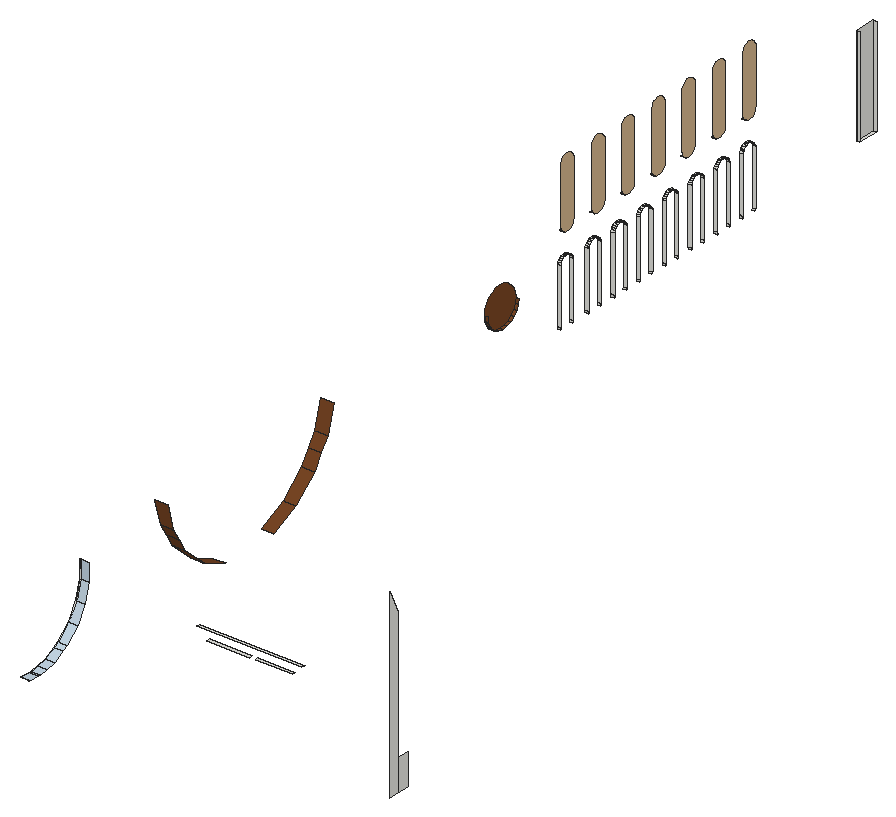
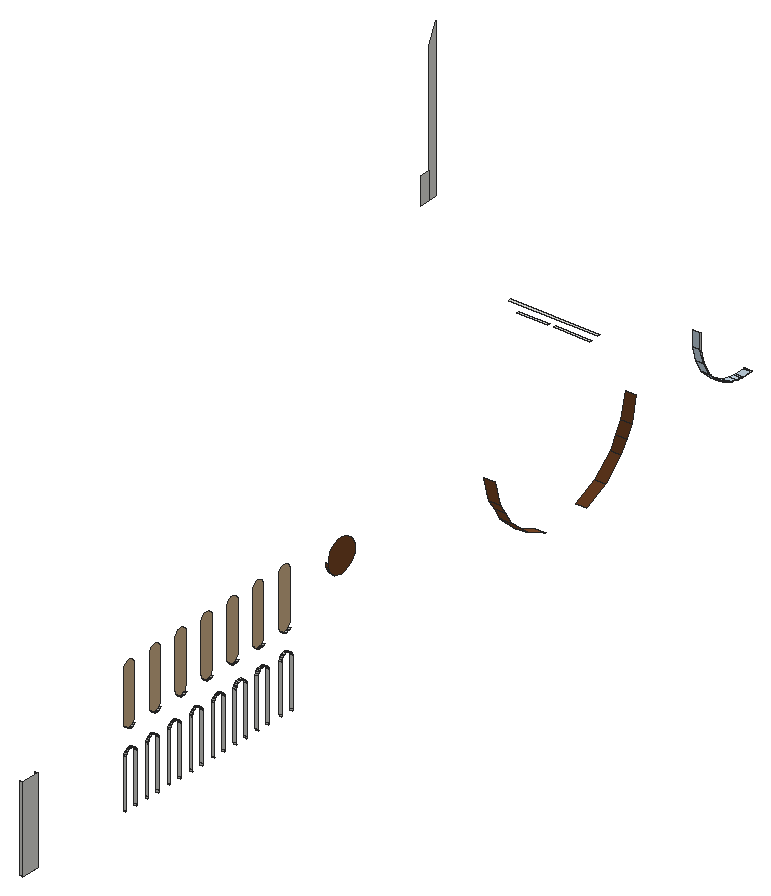
# SketchUp Ruby script. Lengths in inches.
U = 1.inch
M = Sketchup.active_model
def pt(a) = Geom::Point3d.new(a.map { |v| v * U })
def face(e, loops, mat)
  f = e.add_face(loops[0].map { |a| pt(a) })
  loops[1..].each { |l| e.add_face(l.map { |a| pt(a) }).erase! }
  f.material = f.back_material = mat if mat
  f
end
# faces: each face lists its corners as indices into pts; further lists are holes
def faces(e, pts, list, mat = nil) = list.each { |f| face(e, (f[0].is_a?(Array) ? f : [f]).map { |l| l.map { |i| pts[i] } }, mat) }
# xy, xz, yz: faces in a plane at the given z, y or x. An outline is a flat list of corners, or four numbers for a rectangle; further outlines are holes
def ring(l) = l.size == 4 ? [[l[0], l[1]], [l[2], l[1]], [l[2], l[3]], [l[0], l[3]]] : l.each_slice(2).to_a
def flat(e, list, mat, &to3) = list.each { |f| face(e, (f[0].is_a?(Array) ? f : [f]).map { |l| ring(l).map { |u, v| to3.(u, v) } }, mat) }
def xy(e, z, list, mat = nil) = flat(e, list, mat) { |x, y| [x, y, z] }
def xz(e, y, list, mat = nil) = flat(e, list, mat) { |x, z| [x, y, z] }
def yz(e, x, list, mat = nil) = flat(e, list, mat) { |y, z| [x, y, z] }
def lines(e, pts, list) = list.each { |a, b| e.add_line(pt(pts[a]), pt(pts[b])) }
# prism: a flat outline (further loops are holes) pulled along v
def prism(e, loops, v, mat = nil)
  f = face(e, loops, mat); d = Geom::Vector3d.new(v.map { |x| x * U })
  f.pushpull(f.normal.samedirection?(d) ? d.length : -d.length)
end
def box(e, o, s, mat = nil) = prism(e, [[o, [o[0] + s[0], o[1], o[2]], [o[0] + s[0], o[1] + s[1], o[2]], [o[0], o[1] + s[1], o[2]]]], [0, 0, s[2]], mat)
def at(x, y, z, deg = 0) = Geom::Transformation.translation(pt([x, y, z])) * Geom::Transformation.rotation(ORIGIN, Z_AXIS, deg.degrees)
def axes(o, x, y, z) = Geom::Transformation.new([*x, 0, *y, 0, *z, 0, *pt(o).to_a, 1])
def part(name) = M.definitions.add(name)
# library, detail: a bought-in or finely detailed component or shape, given as its bounding box
def library(name, o, s) = part(name).tap { |d| box(d.entities, o, s) }
def detail(e, o, s) = box(e.add_group.entities, o, s)
def put(e, d, t, mat = nil) = e.add_instance(d, t).tap { |i| i.material = mat if mat }
def group(e, t, mat = nil) = e.add_group.tap { |g| g.transformation = t; g.material = mat if mat }.entities
root = M.entities
M.materials.add("[0035_Tan]").color = [210, 180, 140]
M.materials.add("[Terrazzo Light Blue]").color = [196, 214, 227]
M.materials.add("[Wood Veneer 01]").color = [120, 70, 37]
xy(root,212.374,[[48.644,1140.889,51.644,1161.639]])
xy(root,264,[[289.364,148.626,253.365,148.687,253.37,151.687,289.369,151.626],[247.364,148.697,205.364,148.769,205.369,151.769,247.369,151.697]])
xy(root,273.492,[[298.856,148.61,298.861,151.61,195.877,151.785,195.872,148.785]])
xz(root,59.446,[[93.831,232.008,102.831,232.0625]])
xz(root,770.738,[[51.644,212.469,54.644,267.594]])
xz(root,786.176,[[51.644,212.469,54.644,267.594]])
xz(root,804.613,[[51.644,212.469,55.144,267.594]])
xz(root,820.051,[[51.644,212.469,55.144,267.594]])
xz(root,836.238,[[51.644,212.469,55.144,267.594]])
xz(root,851.676,[[51.644,212.469,55.144,267.594]])
xz(root,867.863,[[51.644,212.469,54.644,267.594]])
xz(root,883.301,[[51.644,212.469,54.644,267.594]])
xz(root,899.488,[[51.644,212.469,54.644,267.594]])
xz(root,914.926,[[51.644,212.469,54.644,267.594]])
xz(root,931.113,[[51.644,212.469,54.644,267.594]])
xz(root,946.551,[[51.644,212.469,54.644,267.594]])
xz(root,962.738,[[51.644,212.469,54.644,267.594]])
xz(root,978.176,[[51.644,212.469,54.644,267.594]])
xz(root,994.363,[[51.644,212.469,54.644,267.594]])
xz(root,1009.801,[[51.644,212.469,54.644,267.594]])
xz(root,1140.889,[[48.644,212.374,51.644,309.312]])
xz(root,1161.639,[[48.644,212.374,51.644,309.312]])
yz(root,48.644,[[1140.889,212.374,1161.639,309.312]])
yz(root,54.644,[[778.957,294.25,776.959,294.513,775.098,295.284,773.499,296.511,772.272,298.11,771.501,299.971,771.238,301.969,771.238,357.094,771.844,358.745,772.797,360.222,774.052,361.453,775.547,362.379,777.209,362.953,778.957,363.147,780.704,362.953,782.366,362.379,783.861,361.453,785.116,360.222,786.07,358.745,786.676,357.094,786.676,301.969,786.413,299.971,785.642,298.11,784.415,296.511,782.816,295.284,780.955,294.513],[853.332,294.25,851.334,294.513,849.473,295.284,847.874,296.511,846.647,298.11,845.876,299.971,845.613,301.969,845.613,357.094,846.219,358.745,847.172,360.222,848.427,361.453,849.922,362.379,851.584,362.953,853.332,363.147,855.079,362.953,856.741,362.379,858.236,361.453,859.491,360.222,860.445,358.745,861.051,357.094,861.051,301.969,860.788,299.971,860.017,298.11,858.79,296.511,857.191,295.284,855.33,294.513],[890.519,294.25,888.522,294.513,886.66,295.284,885.061,296.511,883.835,298.11,883.064,299.971,882.801,301.969,882.801,357.094,883.406,358.745,884.36,360.222,885.615,361.453,887.11,362.379,888.772,362.953,890.519,363.147,892.267,362.953,893.929,362.379,895.424,361.453,896.679,360.222,897.633,358.745,898.238,357.094,898.238,301.969,897.975,299.971,897.204,298.11,895.977,296.511,894.379,295.284,892.517,294.513],[927.707,294.25,925.709,294.513,923.848,295.284,922.249,296.511,921.022,298.11,920.251,299.971,919.988,301.969,919.988,357.094,920.594,358.745,921.547,360.222,922.802,361.453,924.297,362.379,925.959,362.953,927.707,363.147,929.454,362.953,931.116,362.379,932.611,361.453,933.866,360.222,934.82,358.745,935.426,357.094,935.426,301.969,935.163,299.971,934.392,298.11,933.165,296.511,931.566,295.284,929.705,294.513],[964.894,294.25,962.897,294.513,961.035,295.284,959.436,296.511,958.21,298.11,957.439,299.971,957.176,301.969,957.176,357.094,957.781,358.745,958.735,360.222,959.99,361.453,961.485,362.379,963.147,362.953,964.894,363.147,966.642,362.953,968.304,362.379,969.799,361.453,971.054,360.222,972.008,358.745,972.613,357.094,972.613,301.969,972.35,299.971,971.579,298.11,970.352,296.511,968.754,295.284,966.892,294.513],
  [1002.082,294.25,1000.084,294.513,998.223,295.284,996.624,296.511,995.397,298.11,994.626,299.971,994.363,301.969,994.363,357.094,994.969,358.745,995.922,360.222,997.177,361.453,998.672,362.379,1000.334,362.953,1002.082,363.147,1003.829,362.953,1005.491,362.379,1006.986,361.453,1008.241,360.222,1009.195,358.745,1009.801,357.094,1009.801,301.969,1009.538,299.971,1008.767,298.11,1007.54,296.511,1005.941,295.284,1004.08,294.513]],"[0035_Tan]")
yz(root,55.144,[[816.144,294.25,814.147,294.513,812.285,295.284,810.686,296.511,809.46,298.11,808.689,299.971,808.426,301.969,808.426,357.094,809.031,358.745,809.985,360.222,811.24,361.453,812.735,362.379,814.397,362.953,816.144,363.147,817.892,362.953,819.554,362.379,821.049,361.453,822.304,360.222,823.258,358.745,823.863,357.094,823.863,301.969,823.6,299.971,822.829,298.11,821.602,296.511,820.004,295.284,818.142,294.513]],"[0035_Tan]")
yz(root,94.831,[[646.427,281.171,641.525,281.817,636.958,283.709,633.036,286.718,630.027,290.64,628.135,295.207,627.489,300.109,628.135,305.01,630.027,309.578,633.036,313.5,636.958,316.509,641.525,318.401,646.427,319.046,651.328,318.401,655.896,316.509,659.818,313.5,662.827,309.578,664.719,305.01,665.364,300.109,664.719,295.207,662.827,290.64,659.818,286.718,655.896,283.709,651.328,281.817]],"[Wood Veneer 01]")
yz(root,102.831,[[59.446,232.008,59.451,232.008,59.451,232.152,59.446,232.0625]])
yz(root,473.833,[[37.618,269.226,47.368,269.226,47.368,427.928,37.618,450.147],[47.368,269.226,59.368,300]])
p = [[51.644,771.001,210.471],[51.644,770.738,212.469],[54.644,770.738,212.469],[54.644,771.001,210.471],[51.644,786.176,212.469],[51.644,785.913,210.471],
  [54.644,785.913,210.471],[54.644,786.176,212.469],[51.644,804.876,210.471],[51.644,804.613,212.469],[55.144,804.613,212.469],[55.144,804.876,210.471],
  [51.644,820.051,212.469],[51.644,819.788,210.471],[55.144,819.788,210.471],[55.144,820.051,212.469],[51.644,836.501,210.471],[51.644,836.238,212.469],
  [55.144,836.238,212.469],[55.144,836.501,210.471],[51.644,851.676,212.469],[51.644,851.413,210.471],[55.144,851.413,210.471],[55.144,851.676,212.469],
  [51.644,868.126,210.471],[51.644,867.863,212.469],[54.644,867.863,212.469],[54.644,868.126,210.471],[51.644,883.301,212.469],[51.644,883.038,210.471],
  [54.644,883.038,210.471],[54.644,883.301,212.469],[51.644,899.751,210.471],[51.644,899.488,212.469],[54.644,899.488,212.469],[54.644,899.751,210.471],
  [51.644,914.926,212.469],[51.644,914.663,210.471],[54.644,914.663,210.471],[54.644,914.926,212.469],[51.644,931.376,210.471],[51.644,931.113,212.469],
  [54.644,931.113,212.469],[54.644,931.376,210.471],[51.644,946.551,212.469],[51.644,946.288,210.471],[54.644,946.288,210.471],[54.644,946.551,212.469],
  [51.644,963.001,210.471],[51.644,962.738,212.469],[54.644,962.738,212.469],[54.644,963.001,210.471],[51.644,978.176,212.469],[51.644,977.913,210.471],
  [54.644,977.913,210.471],[54.644,978.176,212.469],[51.644,994.626,210.471],[51.644,994.363,212.469],[54.644,994.363,212.469],[54.644,994.626,210.471],
  [51.644,1009.801,212.469],[51.644,1009.538,210.471],[54.644,1009.538,210.471],[54.644,1009.801,212.469],[85.284,321.471,213.866],[85.413,294.344,226.503],
  [73.414,294.344,226.626],[73.285,321.471,213.988],[85.413,407.82,226.503],[85.284,380.693,213.866],[73.285,380.693,213.988],[73.414,407.82,226.626],
  [85.616,271.976,246.384],[73.617,271.976,246.507],[85.616,430.187,246.384],[73.617,430.187,246.507],[94.144,70.324,231.232],[94.144,73.036,231.038],
  [93.831,73.036,231.038],[93.831,70.324,231.232],[94.331,70.324,231.232],[94.331,73.036,231.038],[102.831,73.036,231.038],[102.831,70.324,231.232],
  [94.144,80.605,232.587],[93.831,80.605,232.587],[94.331,80.605,232.587],[102.831,80.605,232.587],[94.144,59.446,232.008],[93.831,59.446,232.008],
  [94.331,59.446,232.008],[102.831,59.446,232.008],[102.831,59.451,232.008],[102.831,59.446,232.0625],[93.831,59.446,232.0625],[93.831,59.453,232.187],
  [102.831,59.453,232.187],[102.831,59.451,232.152],[94.144,90.199,234.549],[93.831,90.199,234.549],[94.331,90.199,234.549],[102.831,90.199,234.549],
  [94.144,100.428,239.806],[93.831,100.428,239.806],[94.331,100.428,239.806],[102.831,100.428,239.806],[94.144,105.78,242.556],[93.831,105.78,242.556],
  [94.331,105.78,242.556],[102.831,105.78,242.556],[93.831,118.625,254.467],[94.144,118.625,254.467],[94.331,118.625,254.467],[102.831,118.625,254.467],
  [85.752,263.749,259.697],[73.753,263.749,259.819],[85.752,438.414,259.697],[73.753,438.414,259.819],[93.831,127.783,269.401],[94.144,127.783,269.401],
  [94.331,127.783,269.401],[102.831,127.783,269.401],[85.876,256.244,271.841],[73.877,256.244,271.963],[85.876,445.919,271.841],[73.877,445.919,271.963],
  [51.644,770.738,267.594],[51.644,771.344,269.245],[54.644,771.344,269.245],[54.644,770.738,267.594],[51.644,785.57,269.245],[51.644,786.176,267.594],
  [54.644,786.176,267.594],[54.644,785.57,269.245],[51.644,804.613,267.594],[51.644,805.219,269.245],[55.144,805.219,269.245],[55.144,804.613,267.594],
  [51.644,819.445,269.245],[51.644,820.051,267.594],[55.144,820.051,267.594],[55.144,819.445,269.245],[51.644,836.238,267.594],[51.644,836.844,269.245],
  [55.144,836.844,269.245],[55.144,836.238,267.594],[51.644,851.07,269.245],[51.644,851.676,267.594],[55.144,851.676,267.594],[55.144,851.07,269.245],
  [51.644,867.863,267.594],[51.644,868.469,269.245],[54.644,868.469,269.245],[54.644,867.863,267.594],[51.644,882.695,269.245],[51.644,883.301,267.594],
  [54.644,883.301,267.594],[54.644,882.695,269.245],[51.644,899.488,267.594],[51.644,900.094,269.245],[54.644,900.094,269.245],[54.644,899.488,267.594],
  [51.644,914.32,269.245],[51.644,914.926,267.594],[54.644,914.926,267.594],[54.644,914.32,269.245],[51.644,931.113,267.594],[51.644,931.719,269.245],
  [54.644,931.719,269.245],[54.644,931.113,267.594],[51.644,945.945,269.245],[51.644,946.551,267.594],[54.644,946.551,267.594],[54.644,945.945,269.245],
  [51.644,962.738,267.594],[51.644,963.344,269.245],[54.644,963.344,269.245],[54.644,962.738,267.594],[51.644,977.57,269.245],[51.644,978.176,267.594],
  [54.644,978.176,267.594],[54.644,977.57,269.245],[51.644,994.363,267.594],[51.644,994.969,269.245],[54.644,994.969,269.245],[54.644,994.363,267.594],
  [51.644,1009.195,269.245],[51.644,1009.801,267.594],[54.644,1009.801,267.594],[54.644,1009.195,269.245],[51.644,772.297,270.722],[54.644,772.297,270.722],
  [51.644,784.616,270.722],[54.644,784.616,270.722],[51.644,806.172,270.722],[55.144,806.172,270.722],[51.644,818.491,270.722],[55.144,818.491,270.722],
  [51.644,837.797,270.722],[55.144,837.797,270.722],[51.644,850.116,270.722],[55.144,850.116,270.722],[51.644,869.422,270.722],[54.644,869.422,270.722],
  [51.644,881.741,270.722],[54.644,881.741,270.722],[51.644,901.047,270.722],[54.644,901.047,270.722],[51.644,913.366,270.722],[54.644,913.366,270.722],
  [51.644,932.672,270.722],[54.644,932.672,270.722],[51.644,944.991,270.722],[54.644,944.991,270.722],[51.644,964.297,270.722],[54.644,964.297,270.722],
  [51.644,976.616,270.722],[54.644,976.616,270.722],[51.644,995.922,270.722],[54.644,995.922,270.722],[51.644,1008.241,270.722],[54.644,1008.241,270.722],
  [93.831,132.576,286.25],[94.144,132.576,286.25],[94.331,132.576,286.25],[102.831,132.576,286.25],[51.644,773.552,271.953],[54.644,773.552,271.953],
  [51.644,783.361,271.953],[54.644,783.361,271.953],[51.644,807.427,271.953],[55.144,807.427,271.953],[51.644,817.236,271.953],[55.144,817.236,271.953],
  [51.644,839.052,271.953],[55.144,839.052,271.953],[51.644,848.861,271.953],[55.144,848.861,271.953],[51.644,870.677,271.953],[54.644,870.677,271.953],
  [51.644,880.486,271.953],[54.644,880.486,271.953],[51.644,902.302,271.953],[54.644,902.302,271.953],[51.644,912.111,271.953],[54.644,912.111,271.953],
  [51.644,933.927,271.953],[54.644,933.927,271.953],[51.644,943.736,271.953],[54.644,943.736,271.953],[51.644,965.552,271.953],[54.644,965.552,271.953],
  [51.644,975.361,271.953],[54.644,975.361,271.953],[51.644,997.177,271.953],[54.644,997.177,271.953],[51.644,1006.986,271.953],[54.644,1006.986,271.953],
  [86.14,249.3,297.646],[74.14,249.3,297.769],[86.14,452.863,297.646],[74.14,452.863,297.769],[51.644,775.047,272.879],[54.644,775.047,272.879],
  [51.644,781.866,272.879],[54.644,781.866,272.879],[51.644,808.922,272.879],[55.144,808.922,272.879],[51.644,815.741,272.879],[55.144,815.741,272.879],
  [51.644,840.547,272.879],[55.144,840.547,272.879],[51.644,847.366,272.879],[55.144,847.366,272.879],[51.644,872.172,272.879],[54.644,872.172,272.879],
  [51.644,878.991,272.879],[54.644,878.991,272.879],[51.644,903.797,272.879],[54.644,903.797,272.879],[51.644,910.616,272.879],[54.644,910.616,272.879],
  [51.644,935.422,272.879],[54.644,935.422,272.879],[51.644,942.241,272.879],[54.644,942.241,272.879],[51.644,967.047,272.879],[54.644,967.047,272.879],
  [51.644,973.866,272.879],[54.644,973.866,272.879],[51.644,998.672,272.879],[54.644,998.672,272.879],[51.644,1005.491,272.879],[54.644,1005.491,272.879],
  [51.644,776.709,273.453],[54.644,776.709,273.453],[51.644,780.204,273.453],[54.644,780.204,273.453],[51.644,810.584,273.453],[55.144,810.584,273.453],
  [51.644,814.079,273.453],[55.144,814.079,273.453],[51.644,842.209,273.453],[55.144,842.209,273.453],[51.644,845.704,273.453],[55.144,845.704,273.453],
  [51.644,873.834,273.453],[54.644,873.834,273.453],[51.644,877.329,273.453],[54.644,877.329,273.453],[51.644,905.459,273.453],[54.644,905.459,273.453],
  [51.644,908.954,273.453],[54.644,908.954,273.453],[51.644,937.084,273.453],[54.644,937.084,273.453],[51.644,940.579,273.453],[54.644,940.579,273.453],
  [51.644,968.709,273.453],[54.644,968.709,273.453],[51.644,972.204,273.453],[54.644,972.204,273.453],[51.644,1000.334,273.453],[54.644,1000.334,273.453],
  [51.644,1003.829,273.453],[54.644,1003.829,273.453],[51.644,778.457,273.647],[54.644,778.457,273.647],[51.644,812.332,273.647],[55.144,812.332,273.647],
  [51.644,843.957,273.647],[55.144,843.957,273.647],[51.644,875.582,273.647],[54.644,875.582,273.647],[51.644,907.207,273.647],[54.644,907.207,273.647],
  [51.644,938.832,273.647],[54.644,938.832,273.647],[51.644,970.457,273.647],[54.644,970.457,273.647],[51.644,1002.082,273.647],[54.644,1002.082,273.647],
  [97.831,646.427,281.171],[97.831,641.525,281.817],[94.831,641.525,281.817],[94.831,646.427,281.171],[97.831,651.328,281.817],[94.831,651.328,281.817],
  [97.831,636.958,283.709],[94.831,636.958,283.709],[97.831,655.896,283.709],[94.831,655.896,283.709],[97.831,633.036,286.718],[94.831,633.036,286.718],
  [97.831,659.818,286.718],[94.831,659.818,286.718],[93.831,132.649,303.768],[94.144,132.649,303.768],[94.331,132.649,303.768],[102.831,132.649,303.768],
  [97.831,630.027,290.64],[94.831,630.027,290.64],[97.831,662.827,290.64],[94.831,662.827,290.64],[97.831,628.135,295.207],[94.831,628.135,295.207],
  [97.831,664.719,295.207],[94.831,664.719,295.207],[51.644,778.957,294.25],[51.644,776.959,294.513],[54.644,776.959,294.513],[54.644,778.957,294.25],
  [51.644,780.955,294.513],[54.644,780.955,294.513],[51.644,816.144,294.25],[51.644,814.147,294.513],[55.144,814.147,294.513],[55.144,816.144,294.25],
  [51.644,818.142,294.513],[55.144,818.142,294.513],[51.644,853.332,294.25],[51.644,851.334,294.513],[54.644,851.334,294.513],[54.644,853.332,294.25],
  [51.644,855.33,294.513],[54.644,855.33,294.513],[51.644,890.519,294.25],[51.644,888.522,294.513],[54.644,888.522,294.513],[54.644,890.519,294.25],
  [51.644,892.517,294.513],[54.644,892.517,294.513],[51.644,927.707,294.25],[51.644,925.709,294.513],[54.644,925.709,294.513],[54.644,927.707,294.25],
  [51.644,929.705,294.513],[54.644,929.705,294.513],[51.644,964.894,294.25],[51.644,962.897,294.513],[54.644,962.897,294.513],[54.644,964.894,294.25],
  [51.644,966.892,294.513],[54.644,966.892,294.513],[51.644,1002.082,294.25],[51.644,1000.084,294.513],[54.644,1000.084,294.513],[54.644,1002.082,294.25],
  [51.644,1004.08,294.513],[54.644,1004.08,294.513],[51.644,775.098,295.284],[54.644,775.098,295.284],[51.644,782.816,295.284],[54.644,782.816,295.284],
  [51.644,812.285,295.284],[55.144,812.285,295.284],[51.644,820.004,295.284],[55.144,820.004,295.284],[51.644,849.473,295.284],[54.644,849.473,295.284],
  [51.644,857.191,295.284],[54.644,857.191,295.284],[51.644,886.66,295.284],[54.644,886.66,295.284],[51.644,894.379,295.284],[54.644,894.379,295.284],
  [51.644,923.848,295.284],[54.644,923.848,295.284],[51.644,931.566,295.284],[54.644,931.566,295.284],[51.644,961.035,295.284],[54.644,961.035,295.284],
  [51.644,968.754,295.284],[54.644,968.754,295.284],[51.644,998.223,295.284],[54.644,998.223,295.284],[51.644,1005.941,295.284],[54.644,1005.941,295.284],
  [97.831,627.489,300.109],[94.831,627.489,300.109],[97.831,665.364,300.109],[94.831,665.364,300.109],[51.644,773.499,296.511],[54.644,773.499,296.511],
  [51.644,784.415,296.511],[54.644,784.415,296.511],[51.644,810.686,296.511],[55.144,810.686,296.511],[51.644,821.602,296.511],[55.144,821.602,296.511],
  [51.644,847.874,296.511],[54.644,847.874,296.511],[51.644,858.79,296.511],[54.644,858.79,296.511],[51.644,885.061,296.511],[54.644,885.061,296.511],
  [51.644,895.977,296.511],[54.644,895.977,296.511],[51.644,922.249,296.511],[54.644,922.249,296.511],[51.644,933.165,296.511],[54.644,933.165,296.511],
  [51.644,959.436,296.511],[54.644,959.436,296.511],[51.644,970.352,296.511],[54.644,970.352,296.511],[51.644,996.624,296.511],[54.644,996.624,296.511],
  [51.644,1007.54,296.511],[54.644,1007.54,296.511],[102.831,55.662,234.017],[102.831,55.655,233.892],[93.831,55.5625,232.285],[93.831,55.57,232.41],
  [102.831,60.321,233.625],[102.769,60.321,233.625],[102.831,70.435,233.17],[102.769,70.435,233.17],[102.831,70.289,230.611]]
faces(root,p,[[0,1,2,3],[4,5,6,7],[8,9,10,11],[12,13,14,15],[16,17,18,19],[20,21,22,23],[24,25,26,27],[28,29,30,31],
  [32,33,34,35],[36,37,38,39],[40,41,42,43],[44,45,46,47],[48,49,50,51],[52,53,54,55],[56,57,58,59],[60,61,62,63],
  [76,77,78,79],[76,80,81,77],[77,84,85,78],[77,81,86,84],[88,76,79,89],[88,90,80,76],[93,94,95,96,97],[84,98,99,85],
  [84,86,100,98],[98,102,103,99],[98,100,104,102],[102,106,107,103],[102,104,108,106],[110,107,106,111],[106,108,112,111],[118,110,111,119],
  [111,112,120,119],[126,127,128,129],[130,131,132,133],[134,135,136,137],[138,139,140,141],[142,143,144,145],[146,147,148,149],[150,151,152,153],
  [154,155,156,157],[158,159,160,161],[162,163,164,165],[166,167,168,169],[170,171,172,173],[174,175,176,177],[178,179,180,181],[182,183,184,185],
  [186,187,188,189],[127,190,191,128],[192,130,133,193],[135,194,195,136],[196,138,141,197],[143,198,199,144],[200,146,149,201],[151,202,203,152],
  [204,154,157,205],[159,206,207,160],[208,162,165,209],[167,210,211,168],[212,170,173,213],[175,214,215,176],[216,178,181,217],[183,218,219,184],
  [220,186,189,221],[222,118,119,223],[119,120,224,223],[190,226,227,191],[228,192,193,229],[194,230,231,195],[232,196,197,233],[198,234,235,199],
  [236,200,201,237],[202,238,239,203],[240,204,205,241],[206,242,243,207],[244,208,209,245],[210,246,247,211],[248,212,213,249],[214,250,251,215],
  [252,216,217,253],[218,254,255,219],[256,220,221,257],[226,262,263,227],[264,228,229,265],[230,266,267,231],[268,232,233,269],[234,270,271,235],
  [272,236,237,273],[238,274,275,239],[276,240,241,277],[242,278,279,243],[280,244,245,281],[246,282,283,247],[284,248,249,285],[250,286,287,251],
  [288,252,253,289],[254,290,291,255],[292,256,257,293],[262,294,295,263],[296,264,265,297],[266,298,299,267],[300,268,269,301],[270,302,303,271],
  [304,272,273,305],[274,306,307,275],[308,276,277,309],[278,310,311,279],[312,280,281,313],[282,314,315,283],[316,284,285,317],[286,318,319,287],
  [320,288,289,321],[290,322,323,291],[324,292,293,325],[294,326,327,295],[326,296,297,327],[298,328,329,299],[328,300,301,329],[302,330,331,303],
  [330,304,305,331],[306,332,333,307],[332,308,309,333],[310,334,335,311],[334,312,313,335],[314,336,337,315],[336,316,317,337],[318,338,339,319],
  [338,320,321,339],[322,340,341,323],[340,324,325,341],[356,222,223,357],[223,224,358,357],[368,369,370,371],[372,368,371,373],[374,375,376,377],
  [378,374,377,379],[380,381,382,383],[384,380,383,385],[386,387,388,389],[390,386,389,391],[392,393,394,395],[396,392,395,397],[398,399,400,401],
  [402,398,401,403],[404,405,406,407],[408,404,407,409],[369,410,411,370],[412,372,373,413],[375,414,415,376],[416,378,379,417],[381,418,419,382],
  [420,384,385,421],[387,422,423,388],[424,390,391,425],[393,426,427,394],[428,396,397,429],[399,430,431,400],[432,402,403,433],[405,434,435,406],
  [436,408,409,437],[410,442,443,411],[444,412,413,445],[414,446,447,415],[448,416,417,449],[418,450,451,419],[452,420,421,453],[422,454,455,423],
  [456,424,425,457],[426,458,459,427],[460,428,429,461],[430,462,463,431],[464,432,433,465],[434,466,467,435],[468,436,437,469]])
faces(root,p,[[64,65,66,67],[68,69,70,71],[65,72,73,66],[74,68,71,75],[72,114,115,73],[116,74,75,117],[114,122,123,115],[124,116,117,125],
  [122,258,259,123],[260,124,125,261],[342,343,344,345],[346,342,345,347],[343,348,349,344],[350,346,347,351],[348,352,353,349],[354,350,351,355],
  [352,360,361,353],[362,354,355,363],[360,364,365,361],[366,362,363,367],[364,438,439,365],[440,366,367,441]],"[Wood Veneer 01]")
faces(root,p,[[82,81,80,83],[87,86,81,82],[83,80,90,91,92],[101,100,86,87],[105,104,100,101],[109,108,104,105],[113,112,108,109],[121,120,112,113],
  [225,224,120,121],[359,358,224,225]],"[Terrazzo Light Blue]")
lines(root,p,[[470,471],[472,473],[474,475],[476,477],[83,478]])
